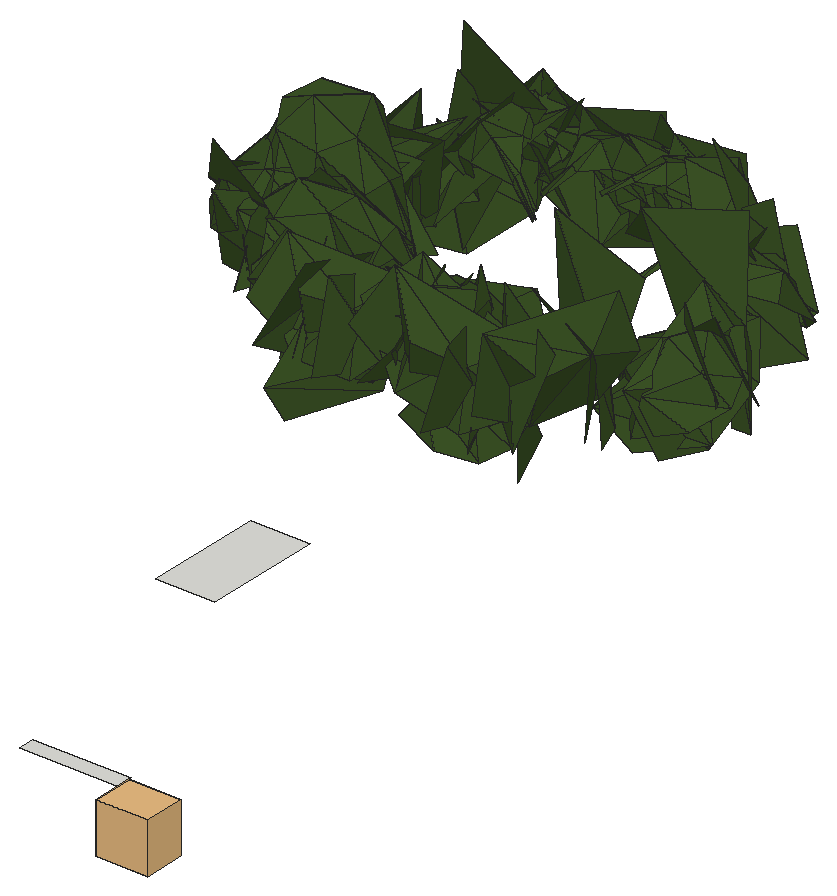
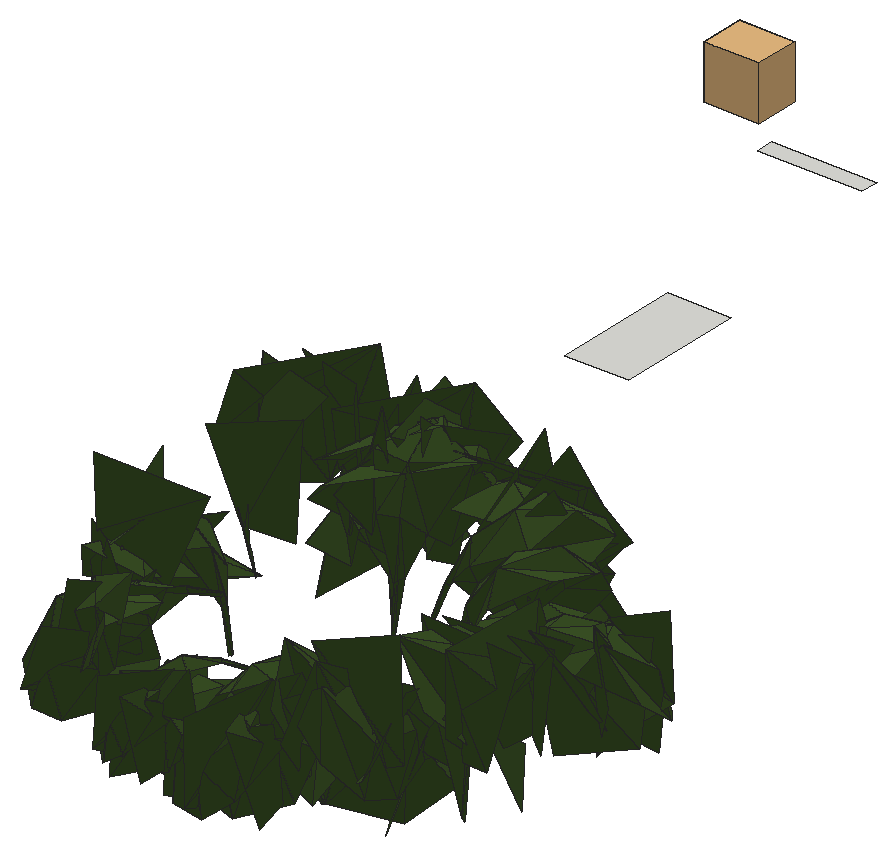
# SketchUp Ruby script. Lengths in inches.
U = 1.inch
M = Sketchup.active_model
def pt(a) = Geom::Point3d.new(a.map { |v| v * U })
def face(e, loops, mat)
  f = e.add_face(loops[0].map { |a| pt(a) })
  loops[1..].each { |l| e.add_face(l.map { |a| pt(a) }).erase! }
  f.material = f.back_material = mat if mat
  f
end
# faces: each face lists its corners as indices into pts; further lists are holes
def faces(e, pts, list, mat = nil) = list.each { |f| face(e, (f[0].is_a?(Array) ? f : [f]).map { |l| l.map { |i| pts[i] } }, mat) }
# xy, xz, yz: faces in a plane at the given z, y or x. An outline is a flat list of corners, or four numbers for a rectangle; further outlines are holes
def ring(l) = l.size == 4 ? [[l[0], l[1]], [l[2], l[1]], [l[2], l[3]], [l[0], l[3]]] : l.each_slice(2).to_a
def flat(e, list, mat, &to3) = list.each { |f| face(e, (f[0].is_a?(Array) ? f : [f]).map { |l| ring(l).map { |u, v| to3.(u, v) } }, mat) }
def xy(e, z, list, mat = nil) = flat(e, list, mat) { |x, y| [x, y, z] }
def xz(e, y, list, mat = nil) = flat(e, list, mat) { |x, z| [x, y, z] }
def yz(e, x, list, mat = nil) = flat(e, list, mat) { |y, z| [x, y, z] }
def lines(e, pts, list) = list.each { |a, b| e.add_line(pt(pts[a]), pt(pts[b])) }
# prism: a flat outline (further loops are holes) pulled along v
def prism(e, loops, v, mat = nil)
  f = face(e, loops, mat); d = Geom::Vector3d.new(v.map { |x| x * U })
  f.pushpull(f.normal.samedirection?(d) ? d.length : -d.length)
end
def box(e, o, s, mat = nil) = prism(e, [[o, [o[0] + s[0], o[1], o[2]], [o[0] + s[0], o[1] + s[1], o[2]], [o[0], o[1] + s[1], o[2]]]], [0, 0, s[2]], mat)
def at(x, y, z, deg = 0) = Geom::Transformation.translation(pt([x, y, z])) * Geom::Transformation.rotation(ORIGIN, Z_AXIS, deg.degrees)
def axes(o, x, y, z) = Geom::Transformation.new([*x, 0, *y, 0, *z, 0, *pt(o).to_a, 1])
def part(name) = M.definitions.add(name)
# library, detail: a bought-in or finely detailed component or shape, given as its bounding box
def library(name, o, s) = part(name).tap { |d| box(d.entities, o, s) }
def detail(e, o, s) = box(e.add_group.entities, o, s)
def put(e, d, t, mat = nil) = e.add_instance(d, t).tap { |i| i.material = mat if mat }
def group(e, t, mat = nil) = e.add_group.tap { |g| g.transformation = t; g.material = mat if mat }.entities
root = M.entities
M.materials.add("AM113_062_Tilia").color = [58, 81, 37]
c1 = library("Plante \#58",[-0.43,-1.58,0],[20.84,18.06,17.59])
xy(root,457.89,[[496.21,121.6875,613.65,141.4375]])
xy(root,481.27,[[418.81,422.72,490.37,567.03]])
p = [[540.97,976.49,485.11],[586.99,972.76,427.11],[584.3125,1052.8,402.97],[584,1026.04,484.06],[572.48,1080.04,507.89],[578.02,1117.79,442.6],
  [607.66,1086.25,411.79],[575.2,1097.73,403.14],[534.37,1141.2,498.26],[105.24,1194.14,425.47],[121.625,1168.47,404.47],[161.48,1107,479.16],
  [175.375,1197.67,407.3125],[146.77,1151.76,433.22],[148.65,1204.82,487.21],[206.27,1265.1,435.07],[482.24,889.78,515.23],[489.48,882.64,408.15],
  [460.95,954.53,416.66],[505.1875,1265,495.33],[477.46,1159.64,529.97],[556.16,1237.07,408.72],[515.61,1162.88,412.62],[116.25,1155.61,503.81],
  [88.94,1129.8,409.31],[132.79,1070.9,436.62],[270.03,1280.875,410.51],[208.25,1271.54,454.14],[239.1,1306.7,507.43],[287.65,1323.01,474.2],
  [346.92,1306.79,499.97],[341.16,1318.84,419.95],[202.91,921.375,524.11],[178.74,911.5,421.625],[240.36,957.91,410.57],[226.11,1031.88,479.77],
  [352.42,1248.81,501.53],[354.88,1300.82,439.02],[276.72,1302.08,411.2],[300.3,1300.82,491.83],[209.65,1298.96,448.97],[246.84,1296.92,513.43],
  [546.34,1142.1,528.125],[608.72,1085.8,502.12],[151.55,1215.79,412.06],[132.38,1165.1,434.07],[160.59,1201.06,496.57],[189.85,1279.91,447.7],
  [213.07,922.26,413.75],[260.45,918.83,444.32],[219.03,953.29,484.51],[146.53,954.5,424.43],[383.25,948.27,480.84],[453.94,1081.94,416.67],
  [476.23,1060.37,454.4],[472.4,1065.68,457.83],[450.9375,1083.38,420.04],[493.08,990.7,444.18],[560.16,966.91,428.22],[598.47,1039.36,417.67],
  [554.87,1022.51,481.14],[559.71,1076.31,504.78],[601.29,1106.96,457.59],[474.35,1070.86,454.28],[454.625,1084.51,418.21],[239.9,810.02,455.3],
  [254.3,824.73,418.67],[319.87,890.17,444.88],[93.47,996.51,419.15],[111.89,950.2,445.67],[74.83,983.71,495.54],[61.625,1058.71,442.37],
  [119.64,1221.89,523.38],[143.48,1253.52,419.85],[183.89,1180.96,421.76],[529.18,1269.46,420.04],[517.99,1265.2,468.17],[540.65,1219.86,507.91],
  [559.23,1244.56,447.95],[493.65,1271.78,420.78],[420.01,1235.08,455.8],[461.27,1256.21,477.04],[360.875,1246.85,522.81],[357.71,1269.1,425.31],
  [396.9375,1324.08,421.59],[387.85,1331.93,511.8125],[238.8125,1180.16,527.97],[169.58,978.83,500.55],[157.8125,1052.92,506.86],[105.71,1004.54,490.37],
  [66.62,989.34,425.16],[93.85,947.16,447.4],[84.62,990.76,503.43],[41.61,1055.43,455.22],[538.94,1273.09,438.28],[526.01,1242.08,425.31],
  [445.83,1218.16,482.9],[161.33,1110.96,511.88],[132.95,1191.07,506.82],[252.93,1342.04,524.91],[229.51,1323.07,426.08],[210.26,1259.43,474.66],
  [417.6875,1284.625,504.09],[420.8,1296.35,439.53],[355.75,1299.97,428.5],[384,1321.07,482.25],[307.83,1318.91,461.87],[342.61,1329.74,507.26],
  [397.16,1242.04,503.24],[422.28,1277.85,454.65],[369.27,1311.87,430.07],[383.03,1300.15,496.01],[343.73,1319.63,511.95],[320.43,1337.42,458.78],
  [332.11,1310.22,486.05],[347.19,1290.81,453.34],[314,1340.01,431.26],[271.63,1351.47,433.65],[46.55,973.26,531.23],[34.23,1005.09,432.75],
  [111.03,993.85,432.13],[145.22,1037.9375,527.26],[560.16,939.93,466.21],[538.29,947.72,432.3],[477.78,1017.81,458.78],[285.48,1358.35,443.64],
  [279.97,1325.34,432.66],[249.55,1273.02,524.38],[469.7,830.77,460.16],[452.16,852.8,433.17],[438.91,938.69,482.17],[154.66,1142.45,506.9],
  [284.13,1343.11,479.49],[243.91,1340.17,457.21],[190.08,1129.09,473.03],[345.56,987.98,434.33],[346.28,973.38,485.99],[348.93,979.89,485.06],
  [510.04,1023.32,438.11],[548.59,978.53,434.33],[554.47,988.6,478.09],[607.44,992.39,455.93],[345.54,992.1,435.5625],[353.67,979.48,479.96],
  [348.24,989.09,434.62],[164.39,1261.91,512.26],[205,1275.19,584.18],[205.57,1323.22,520.33],[234.72,1045.24,468.94],[243.37,1069.75,435.25],
  [244.5,1072.77,438.52],[241.07,1071.49,435.79],[225.32,1046.33,475.27],[232.31,1047.3,475.79],[215.23,1104.59,460.99],[498.43,1033.25,470.35],
  [436.38,1233.07,507.66],[506.33,1283.28,517.15],[366.5625,1348.27,523.18],[344.91,1346.09,441.6875],[303.62,1309.42,478.09],[42,1028.72,517.38],
  [56.84,1068.96,581.47],[20.07,1094.33,521.55],[563.75,1142.42,501.66],[401.08,850.02,493.5625],[435.85,821.7,450.7],[475.93,840.39,442.99],
  [459.9,854.41,485.42],[489.22,873.06,449.4375],[350.56,980.44,443.21],[369.27,952.11,476.46],[370.12,958.83,479.09],[350.1,983.51,446.91],
  [372.98,961.76,473.12],[352.85,982.24,443.34],[247.76,1282.89,554.875],[289.59,1354.88,532.32],[510.76,1132.38,497.6875],[283.41,983.85,455.9],
  [251.84,1198.38,551.67],[247.12,1263.74,444.81],[174.92,1315.79,466.3],[324.41,897.16,476.76],[124.97,953.45,513.89],[154.19,970.84,479.86],
  [188.24,1248.09,531.9],[261.4375,1247.36,574.97],[225.83,1311.42,543.21],[557.79,1191.3125,490.71],[139.65,1058.8,548.31],[86.03,1088.53,448.54],
  [6.96,1065.44,473.4],[398.09,1346.88,458.79],[380.72,1326.41,448.45],[335.31,1301.77,519.97],[409.2,1293.38,492.54],[412.38,1273.96,465.67],
  [410.53,1322.32,448.8],[385.85,1348.04,450.06],[185.73,1294.63,508.65],[467.85,911.13,495.71],[470.62,956.12,470.29],[262.77,947.97,550.35],
  [241.75,891.36,449.65],[222.5625,816.03,492.71],[442.9,1187.43,536.27],[455.72,1227.375,450.13],[512.02,1262.72,465.91],[389.84,1336.44,487.22],
  [361.26,1351.55,467.98],[377.23,842.77,460.3],[331.33,961.08,504.57],[363.43,877.625,450.67],[380.8125,826.86,535.04],[588.11,1056.17,545.74],
  [558.97,1121.25,450.95],[487.97,1063.12,465.68],[623.71,1078.44,452.45],[625.65,1014.33,483.85],[606.33,1029.9,451.87],[535.36,1082.41,496.55],
  [136.99,1139.08,452.6],[136.57,1068.125,457.15],[112.18,1082.83,528.78],[103.82,1139.54,528.08],[133.4,1181.28,579],[115,1204.74,506.74],
  [317.43,1248.61,488.12],[184.61,1277.3,515],[81.71,1094.41,559.34],[88.7,1103.95,454.24],[150.2,1061.27,474.03],[502.01,1051.02,496.8125],
  [516.53,1074.43,498.88],[201.59,1129.52,569.22],[171.79,1154.85,454.48],[91.7,1175.35,467.63],[215.72,940.66,499.76],[254.03,949.51,461.64],
  [233.1,989.79,455.05],[233.56,993.77,492.58],[66.23,1039.24,534.09],[109.29,1094.59,569.02],[40.85,1103.46,541.52],[256.01,856.28,519.88],
  [442.73,1196.76,468.87],[629.07,1029.21,472.64],[134.4,917.52,488.71],[145.68,939.95,457.11],[231.67,975.67,480.33],[130.35,1027.53,500.52],
  [213.27,1278.82,522.65],[247.03,1313.48,520.05],[579.73,1135.16,508.51],[426.61,948.19,458.24],[421.46,943.03,494.93],[477.0625,1028.125,489.66],
  [337.41,1309.01,545.03],[397.21,1341.71,530.66],[300.46,1343.76,506.36],[109.77,1075.1,459.125],[113.23,1033.17,499.13],[123.7,1086.28,536.15],
  [117.71,1147.9,461.3],[215.49,1055.25,504.9375],[222.41,1064.02,459.65],[226.3,1065.19,460.36],[446.26,943.62,513.8125],[462.53,861.38,540.89],
  [222.4375,1066.9,460.15],[213.42,1063.21,513.69],[218.2,1058.55,510.7],[371.3,901.625,462.21],[129.23,1141.65,545.81],[191.17,1177.21,570.87],
  [136.67,1207.93,527.23],[177.14,909.64,464.61],[292.26,1332.11,510.8],[258.7,857.78,462.09],[256.52,843.22,548.15],[211.68,882.2,584.12],
  [313.8125,853.61,548.08],[190.82,846.63,520.23],[330.54,861.1,469.81],[129.21,1253.68,462.15],[158.58,1165.8,466.8125],[144.07,1206.09,506.3125],
  [142.93,1267.27,518.4],[137.19,1289.91,473.46],[378.01,918.12,492.22],[261.98,1010.71,528.54],[186.7,972.22,462.88],[129.93,951.41,539.22],
  [296.14,998.26,463.17],[276.98,996.66,512.25],[283.71,994.5,512.37],[300.11,998.59,465.02],[388.14,845.65,480.83],[457.46,860.53,463.5],
  [460.9375,840.51,540.95],[505.34,867.18,494.3],[284.12,989.72,507.33],[297.42,995.67,463.68],[510.62,1203.77,531.68],[522.87,1225.59,473.625],
  [464.63,1255.09,463.96],[494.07,1253.09,523.2],[456.71,1271.36,550.1],[424.2,1283.36,502.46],[141.92,913.85,468.79],[158.61,933.4,506.95],
  [373.14,1256.75,491.43],[499.14,1255.65,555.46],[527.42,968.33,537.18],[142.82,1248.15,541.83],[203.41,1181.16,482.35],[91.27,1127.79,562.29],
  [312.6,1321.05,517.83],[350.625,1330.97,517.97],[482.76,1233.98,511.35],[243.73,1232.38,572.18],[177.04,1241.07,468.25],[103.2,1277.62,514.84],
  [140.84,989.09,519.9],[115.48,947.72,484.33],[219.62,1013.45,509.875],[446.46,1206.21,504.42],[526.42,1089.61,469.06],[569.76,1071.03,522.16],
  [552.36,1115.03,504.79],[476.46,1173.45,515.92],[516.4375,1205.57,481.74],[481.3,1260.42,469.68],[484.61,1232.07,529.15],[453.77,1260.99,551.1],
  [442.74,1295.84,506],[370.41,866.71,516.0625],[385.58,825.66,494.03],[457.3,832.84,470.26],[456.16,851.875,548.125],[503.65,848.99,496.37],
  [544.08,1039.8,515.21],[598.59,1023.05,503.4],[618.94,1061.01,488.7],[398.21,932.05,507.875],[26.99,996.17,473.22],[108.95,968.15,476.0625],
  [71.73,981.74,513.67],[25.99,1016.1,524.61],[4.91,1023.07,482.95],[40.65,1006.01,546.6],[196.8125,1275.78,560.28],[169.9375,1311.25,508.875],
  [136.03,1296.34,496.19],[165.93,1281.92,473.59],[182.18,1184.03,501.13],[197.42,1104.92,557.17],[285.02,1230.43,530.29],[198.53,1029.16,500.04],
  [123.35,1010.625,487.24],[175.92,1031.03,476.13],[121.9,1009.9,491.2],[461.96,811.09,577.63],[433.55,805.56,476.43],[463.73,877.06,476.65],
  [424.54,922.73,567.22],[249.96,840.79,477.65],[324.09,835.32,481.86],[309.76,866.37,550.58],[214.61,936.46,553.9],[186.33,872.29,531.5],
  [253.12,871.91,555.34],[341.93,1257.24,524.05],[284.61,1301.19,529.06],[419.16,913.8,606.23],[443.11,864.71,524.55],[441.15,934.17,479.93],
  [356.75,969.11,498.49],[359.5,963.02,536.79],[386.8125,962.68,531.66],[243.9,970.17,509.1875],[319.5,895.38,577.125],[333.6,838.25,543.22],
  [393,867.89,480.61],[383.36,883.18,565.6],[424,924.15,555.53],[447.77,914.87,480.68],[468.46,956.65,515.61],[369.41,845.83,618.59],
  [338.97,815.62,556.53],[408.05,820.35,558.5625],[497.96,818.63,601.05],[501.22,797.55,522.6],[511.3125,872.48,480.89],[542.9375,847.83,552.24],
  [562.52,902.09,562.48],[545.66,934.87,495.96],[0,1026.7,504.2],[27.14,1039.8125,481.07],[109.61,997.23,506.26],[301.8,830.77,589.06],
  [295.52,812.67,484.06],[336.56,878.51,481.16],[288.24,942.04,541.39],[585.15,874.01,587.43],[571.39,880.97,481.41],[537.1875,945.375,515.71],
  [365.17,849.58,521.13],[452.2,1114.74,592.6],[501.0625,1112.5,482.02],[582.59,1110.25,511.01],[196.23,1178.36,521.66],[51.21,1062.35,559.76],
  [8.47,1060.73,513.5],[539.78,1011.5,590.32],[431.99,1009.21,630.39],[519.05,986.28,483.78],[439.25,1009.87,503.42],[530.43,1082.8125,529.58],
  [583.125,1017.34,555.53],[401.84,922.9,586.24],[365.15,876.84,484.07],[366.2,794.92,511.31],[560.75,848.45,586.68],[461.26,897.66,607.9],
  [535.02,817.33,484.64],[472.67,874.51,485.01],[529.34,1113.24,541.26],[430.68,899.86,511.73],[339.23,949.16,521.2],[308.99,1249.99,523.65],
  [122.25,1005.17,524.43],[371.33,1306.56,525.79],[175.84,933.21,558.67],[504.24,1167.18,499.92],[366.9375,1260.83,520.0625],[198.48,973.74,521.03],
  [267.59,839.48,586.71],[358.53,902.82,603.59],[334.28,838.34,575.52],[403.06,846.72,574.14],[501.74,881.75,561.98],[571.82,963.04,544.72],
  [166.49,1170.84,525.57],[125.06,1246.89,567.46],[494.17,913.85,526.3],[161.82,1042.76,520.89],[188.82,1059.52,496.85],[191.37,1060.02,500.95],
  [188.38,1062.18,498.28],[155.32,1048.84,528.44],[160.82,1044.4,528.47],[446.3125,1151.97,513.07],[435.9,1118.375,498.92],[435.32,1116.8,503.75],
  [254,1169.22,522.22],[286.95,1157.31,498.89],[288.82,1155.44,503.42],[175.6,1034.26,535.5],[449.55,1152.5,519.84],[438.34,1117,499.95],
  [456.34,1153.1875,517.47],[484.25,1177.13,524.375],[218.88,1277.07,568.39],[141.16,1040.08,566.46],[254.37,1171.11,530.39],[288.85,1159.4,500.59],
  [254.5625,1178.68,530.43],[400.13,951.74,500.98],[417.34,927.02,571.76],[440.47,954.48,528.39],[210.86,1238.65,547.79],[332.92,924.91,501.63],
  [317.83,873.43,533.82],[335.77,887.8,569.34],[410.52,1291.47,554.11],[293.4375,1293.875,536.58],[314.58,1316.94,554.99],[111.05,979.02,530.26],
  [32.09,993.09,571.79],[463.375,1194.59,528.23],[387.27,899.07,601.23],[203.18,1046.76,562.95],[191.53,1023.03,552.76],[422.64,1299.71,553.92],
  [173.04,1217.61,545.72],[326.12,1288.28,506.6],[339.51,1288.65,531.45],[263.02,982.89,561.35],[265.17,955.62,556.7],[248.14,1252.47,508.93],
  [262.62,1262.27,538.63],[228.58,1293.38,544.22],[337.36,1244.79,527.37],[317.53,1221.39,514.37],[318.71,1222.1,510.38],[341.66,1245.39,522.7],
  [559.38,1144.07,612.63],[333.22,1245.8125,524.15],[316.92,1223.46,511.18],[428.02,813.83,589.86],[249.23,1002,543.38],[55.81,1095.28,542.38],
  [80.53,1011.17,548.28],[197.29,1072.79,555.07],[132.22,1246.73,623.72],[431.58,983.91,553.78],[476.4,918.99,598.91],[395.92,1251.84,565.59],
  [288.22,1214.52,535.05],[281.92,1176.77,521.03],[282.61,1178.12,516.03],[292.25,1217.72,529],[355.15,892.1,575.19],[283.125,1212.85,531.32],
  [279.88,1178.45,517.08],[226.55,1006.4,520.14],[171.49,1017.71,543.97],[183.77,1001.04,581.75],[355.89,1274.49,536.86],[124.4,1024.34,549.89],
  [361.22,918.48,532.02],[376.76,931.05,572.79],[212.63,1188.9,550.28],[150.42,1002.0625,594.38],[162.36,978.06,541.18],[173.56,1020.05,523.04],
  [289.04,1257.96,544.64],[228.42,922.66,591.625],[261.32,901.48,553.18],[258.16,941.39,524.8125],[431.8,872.75,563.75],[121.8,1051.58,548.85],
  [195.8,950.66,616.07],[110.02,1073.79,529.45],[234.09,1208.84,550.96],[246.22,1233.39,531.27],[422.29,1261.07,591.46],[365.16,840.44,565.61],
  [94.57,1010.39,596.89],[147.07,1090.77,617.28],[176.02,1090.68,543.15],[138.03,1118.14,589.73],[229.3125,963.43,592.52],[139.4,968.16,571.35],
  [558,949.28,610.47],[170.37,1037.11,602.26],[176.49,904.125,575.66],[409.44,845.33,569.02],[392,876.79,589.08],[147.2,924.38,576.3],
  [175.21,944.22,600.69],[91.92,1082.33,619.38],[116.35,1040.75,628.21],[79,1039.91,612.95]]
faces(root,p,[[0,1,2],[2,3,0],[4,3,2],[2,5,4],[6,7,8],[9,10,11],[12,13,14],[15,12,14],
  [16,17,18],[19,20,21],[20,22,21],[23,24,25],[26,27,28],[28,29,26],[30,31,26],[26,29,30],
  [32,33,34],[32,34,35],[36,37,38],[38,39,36],[38,40,41],[41,39,38],[42,43,6],[8,42,6],
  [44,45,46],[47,44,46],[48,49,50],[51,48,50],[16,18,52],[53,54,55],[55,56,53],[57,58,59],
  [59,60,57],[61,60,59],[59,62,61],[63,64,56],[65,66,67],[68,69,70],[71,68,70],[72,73,74],
  [56,55,63],[75,76,77],[77,78,75],[75,79,76],[79,80,81],[76,79,81],[82,83,84],[85,82,84],
  [72,74,86],[50,87,51],[88,89,51],[51,87,88],[90,91,92],[93,90,92],[94,95,96],[11,97,9],
  [97,98,9],[99,100,101],[102,103,104],[104,105,102],[104,106,107],[107,105,104],[108,109,110],[110,111,108],
  [112,111,110],[110,113,112],[114,115,116],[114,116,117],[118,119,120],[118,120,121],[122,123,124],[125,126,127],
  [128,129,130],[14,13,131],[117,132,114],[117,133,132],[46,45,134],[135,136,137],[138,139,140],[140,139,141],
  [137,142,135],[143,144,142],[14,145,15],[15,145,146],[146,147,15],[148,149,150],[142,137,143],[151,152,153],
  [153,150,151],[23,25,154],[140,155,138],[96,156,94],[156,157,94],[150,153,148],[158,159,160],[70,161,71],
  [71,161,162],[162,163,71],[5,164,4],[165,166,167],[167,168,165],[167,169,168],[170,171,172],[172,173,170],
  [174,175,173],[127,176,125],[176,177,125],[61,178,57],[57,60,61],[50,49,179],[180,181,182],[67,183,65],
  [70,69,184],[173,172,174],[92,91,185],[46,186,47],[47,186,187],[187,188,47],[77,189,78],[190,191,192],
  [193,194,195],[196,197,198],[196,198,199],[40,200,41],[168,169,201],[169,202,201],[203,204,205],[206,207,208],
  [199,209,196],[199,210,209],[165,211,166],[212,213,214],[215,216,217],[215,218,216],[219,220,221],[222,223,224],
  [224,225,222],[222,225,226],[226,227,222],[228,115,114],[27,229,28],[230,231,232],[63,55,233],[233,234,63],
  [54,155,233],[233,55,54],[235,236,237],[238,239,240],[240,241,238],[92,242,93],[93,242,243],[243,244,93],
  [183,245,65],[81,80,246],[50,179,88],[140,141,247],[248,249,250],[223,251,224],[133,252,253],[132,133,253],
  [62,254,61],[255,256,201],[201,202,255],[124,257,122],[195,258,193],[258,259,193],[113,260,112],[261,262,263],
  [264,261,263],[265,266,267],[130,268,128],[268,269,128],[270,271,272],[272,267,270],[273,211,165],[267,272,265],
  [263,274,264],[264,274,275],[275,276,264],[277,239,238],[106,278,107],[279,280,281],[282,280,279],[281,283,279],
  [279,284,282],[285,286,287],[288,285,287],[289,285,288],[165,290,273],[291,292,293],[294,295,296],[296,297,294],
  [298,299,300],[299,301,300],[302,303,297],[304,305,306],[306,307,304],[308,307,306],[306,309,308],[310,277,311],
  [311,277,238],[297,296,302],[312,197,196],[313,206,208],[257,314,122],[315,180,182],[287,286,316],[317,235,237],
  [210,318,319],[209,210,319],[77,76,320],[321,322,323],[320,76,81],[324,325,310],[310,311,324],[326,241,148],
  [148,153,326],[246,327,81],[328,234,329],[329,330,328],[331,332,333],[333,334,331],[335,334,333],[333,336,335],
  [284,337,282],[338,339,340],[339,341,340],[155,140,342],[342,233,155],[247,343,140],[247,344,343],[46,134,187],
  [174,172,345],[345,256,174],[346,347,348],[349,346,348],[350,346,349],[351,190,192],[289,288,352],[352,353,289],
  [354,355,356],[230,232,357],[30,29,28],[99,101,358],[152,359,326],[326,153,152],[348,347,360],[361,362,324],
  [324,359,361],[363,364,365],[171,290,345],[345,172,171],[363,365,366],[320,81,327],[367,368,369],[370,371,367],
  [367,372,370],[369,372,367],[140,343,342],[158,160,373],[374,132,253],[114,132,374],[375,376,377],[375,377,378],
  [92,185,243],[379,380,143],[143,137,379],[250,381,248],[382,383,384],[384,385,382],[386,385,384],[384,387,386],
  [387,388,386],[389,390,298],[298,391,389],[300,391,298],[392,393,394],[394,395,392],[396,395,394],[394,397,396],
  [398,399,400],[401,402,403],[401,403,404],[405,406,407],[368,408,369],[409,410,411],[102,105,107],[316,412,287],
  [350,349,413],[413,414,350],[415,416,417],[416,418,417],[221,419,219],[419,420,219],[421,422,423],[0,3,4],
  [324,362,325],[88,87,50],[424,425,426],[425,427,426],[379,137,136],[4,428,0],[165,168,429],[429,168,201],
  [136,430,379],[114,431,228],[431,114,374],[360,432,348],[14,131,146],[146,145,14],[196,209,433],[433,209,319],
  [381,434,248],[343,344,329],[344,330,329],[435,189,77],[196,436,312],[36,39,41],[290,165,429],[429,345,290],
  [436,196,433],[437,238,241],[437,241,326],[438,203,205],[439,440,338],[338,441,439],[340,441,338],[300,301,442],
  [429,256,345],[429,201,256],[70,184,162],[162,161,70],[397,443,396],[108,111,112],[444,445,354],[356,444,354],
  [340,341,446],[187,186,46],[342,234,233],[447,448,449],[61,254,178],[450,451,452],[452,449,450],[342,329,234],
  [453,454,455],[456,457,458],[263,262,459],[437,311,238],[460,455,461],[461,462,460],[77,463,435],[359,324,437],
  [437,326,359],[28,464,30],[224,251,465],[466,458,467],[467,468,466],[449,452,447],[469,380,470],[470,471,469],
  [41,472,36],[473,474,475],[475,430,473],[4,164,428],[309,476,308],[112,477,108],[243,242,92],[342,343,329],
  [458,466,456],[455,460,453],[107,478,102],[400,479,398],[479,480,398],[481,327,453],[320,327,481],[482,212,214],
  [483,484,265],[265,272,483],[336,485,335],[486,287,412],[486,288,287],[112,260,477],[319,318,487],[487,488,319],
  [324,311,437],[489,490,302],[302,296,489],[107,278,478],[28,229,464],[463,77,320],[41,200,472],[253,252,491],
  [491,492,253],[352,493,353],[494,495,496],[496,497,494],[483,272,271],[498,409,411],[499,500,495],[501,421,423],
  [320,481,463],[295,502,489],[489,296,295],[453,460,481],[413,503,414],[504,349,348],[504,348,432],[271,505,483],
  [495,494,499],[506,321,323],[386,388,507],[405,407,508],[335,509,331],[331,334,335],[510,511,512],[512,513,510],
  [282,337,514],[515,516,511],[481,460,462],[462,463,481],[433,319,488],[352,288,486],[374,253,492],[517,518,519],
  [519,502,517],[497,436,520],[433,520,436],[521,432,447],[447,452,521],[511,510,515],[369,408,522],[430,475,523],
  [523,379,430],[524,412,456],[486,412,524],[456,466,524],[520,494,497],[525,526,527],[527,484,525],[304,307,308],
  [513,431,528],[374,528,431],[499,494,520],[520,488,499],[504,432,521],[413,349,504],[529,530,531],[531,490,529],
  [433,488,520],[340,446,439],[226,225,224],[532,471,470],[451,533,521],[521,452,451],[534,291,293],[224,465,226],
  [528,510,513],[374,492,528],[413,533,535],[535,503,413],[524,466,468],[468,536,524],[352,536,537],[528,492,515],
  [515,510,528],[537,493,352],[523,470,380],[523,380,379],[308,538,304],[369,522,370],[475,474,539],[263,459,275],
  [275,274,263],[389,391,300],[300,442,389],[540,526,525],[541,505,542],[542,543,541],[502,519,544],[544,489,502],
  [519,518,545],[396,443,546],[486,524,536],[536,352,486],[281,280,282],[439,441,340],[282,514,281],[533,413,504],
  [504,521,533],[308,476,538],[370,372,369],[335,485,509],[392,395,396],[547,525,484],[547,484,483],[548,530,529],
  [386,507,382],[505,541,547],[547,483,505],[382,385,386],[544,529,490],[544,490,489],[396,546,392],[549,532,550],
  [550,532,470],[475,539,549],[549,550,475],[475,550,523],[519,545,551],[523,550,470],[551,548,552],[552,548,529],
  [551,552,519],[519,552,544],[541,543,553],[544,552,529],[554,540,525],[547,554,525],[555,540,554],[541,554,547],
  [541,553,555],[555,554,541]],"AM113_062_Tilia")
put(root,c1,axes([663.81,32.98,439.71],[2.9928,0,0],[0,2.7666,0],[0,0,3.48]))
